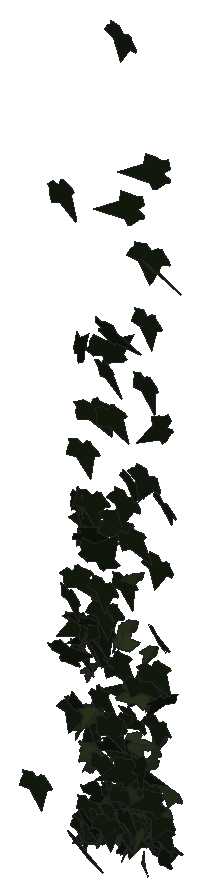
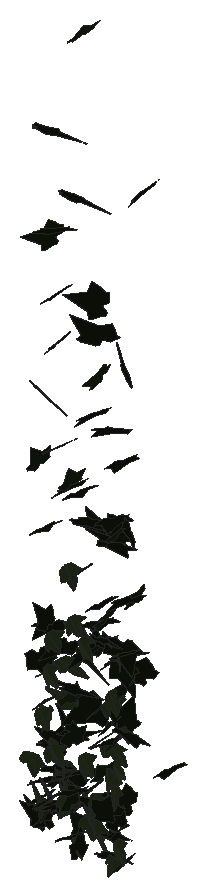
# SketchUp Ruby script. Lengths in inches.
U = 1.inch
M = Sketchup.active_model
def pt(a) = Geom::Point3d.new(a.map { |v| v * U })
def face(e, loops, mat)
  f = e.add_face(loops[0].map { |a| pt(a) })
  loops[1..].each { |l| e.add_face(l.map { |a| pt(a) }).erase! }
  f.material = f.back_material = mat if mat
  f
end
# faces: each face lists its corners as indices into pts; further lists are holes
def faces(e, pts, list, mat = nil) = list.each { |f| face(e, (f[0].is_a?(Array) ? f : [f]).map { |l| l.map { |i| pts[i] } }, mat) }
# xy, xz, yz: faces in a plane at the given z, y or x. An outline is a flat list of corners, or four numbers for a rectangle; further outlines are holes
def ring(l) = l.size == 4 ? [[l[0], l[1]], [l[2], l[1]], [l[2], l[3]], [l[0], l[3]]] : l.each_slice(2).to_a
def flat(e, list, mat, &to3) = list.each { |f| face(e, (f[0].is_a?(Array) ? f : [f]).map { |l| ring(l).map { |u, v| to3.(u, v) } }, mat) }
def xy(e, z, list, mat = nil) = flat(e, list, mat) { |x, y| [x, y, z] }
def xz(e, y, list, mat = nil) = flat(e, list, mat) { |x, z| [x, y, z] }
def yz(e, x, list, mat = nil) = flat(e, list, mat) { |y, z| [x, y, z] }
def lines(e, pts, list) = list.each { |a, b| e.add_line(pt(pts[a]), pt(pts[b])) }
# prism: a flat outline (further loops are holes) pulled along v
def prism(e, loops, v, mat = nil)
  f = face(e, loops, mat); d = Geom::Vector3d.new(v.map { |x| x * U })
  f.pushpull(f.normal.samedirection?(d) ? d.length : -d.length)
end
def box(e, o, s, mat = nil) = prism(e, [[o, [o[0] + s[0], o[1], o[2]], [o[0] + s[0], o[1] + s[1], o[2]], [o[0], o[1] + s[1], o[2]]]], [0, 0, s[2]], mat)
def at(x, y, z, deg = 0) = Geom::Transformation.translation(pt([x, y, z])) * Geom::Transformation.rotation(ORIGIN, Z_AXIS, deg.degrees)
def axes(o, x, y, z) = Geom::Transformation.new([*x, 0, *y, 0, *z, 0, *pt(o).to_a, 1])
def part(name) = M.definitions.add(name)
# library, detail: a bought-in or finely detailed component or shape, given as its bounding box
def library(name, o, s) = part(name).tap { |d| box(d.entities, o, s) }
def detail(e, o, s) = box(e.add_group.entities, o, s)
def put(e, d, t, mat = nil) = e.add_instance(d, t).tap { |i| i.material = mat if mat }
def group(e, t, mat = nil) = e.add_group.tap { |g| g.transformation = t; g.material = mat if mat }.entities
root = M.entities
M.materials.add("1026 AP 7946 SUNNY SIDE UP").color = [254, 231, 186]
M.materials.add("efeu1").color = [18, 25, 13]
M.materials.add("efeu2").color = [43, 57, 29]
c1 = part("ivyleaf_9")
p = [[1.54,2.16,1.25],[1.36,2.04,1.19],[-0.21,0.99,0.68],[-0.71,1.11,0.82],[-0.85,0.86,0.67],[-0.8,0.17,0.21],
  [-0.9,-0.01,0.1],[-0.67,-0.16,-0.02],[-0.08,-0.08,-0.05],[-0.03,-0.6,-0.4],[0.65,-0.88,-0.66],[0.83,-0.6,-0.49],
  [1.29,-0.42,-0.43],[1.8125,-0.07,-0.26],[1.21,0.44,0.15]]
faces(c1.entities,p,[[0,1,2,3,4,5,6,7,8,9,10,11,12,13,14]],"efeu1")
c2 = part("ivyleaf_10")
p = [[0,0.5,-0.03],[-0.0625,2.02,-0.43],[-0.19,2.01,-0.46],[-0.54,1.05,-0.29],[-0.52,0.625,-0.18],[-0.83,0.76,-0.28],
  [-1.16,0.64,-0.33],[-1.15,0.33,-0.24],[-0.77,-0.39,0.02],[-0.3,-0.51,0.16],[0.04,-0.48,0.23],[-0.02,2.01,-0.4375],
  [-0.06,2.01,-0.43],[0.04,-0.49,0.23],[0.67,-0.49,0.14],[1.38,0.36,-0.2],[1.375,0.51,-0.24],[0.81,0.65,-0.19],
  [0.62,0.59,-0.15],[0.6,1.09,-0.28],[0.5,1.23,-0.31]]
faces(c2.entities,p,[[0,1,2,3,4,5,6,7,8,9,10],[11,12,0,13,14,15,16,17,18,19,20]],"efeu2")
put(root,c1,axes([128.56,209.27,294.41],[-0.04738,-0.42398,-0.02706],[0.01155,0.0234,-0.4377],[0.66762,-0.03049,0.00565]),"1026 AP 7946 SUNNY SIDE UP")
put(root,c1,axes([128.95,211.87,300.18],[-0.0411,0.3727,-0.15385],[0.00882,-0.15142,-0.38575],[-0.63252,-0.02633,0.00462]),"1026 AP 7946 SUNNY SIDE UP")
put(root,c1,axes([128.49,211.98,306.7],[-0.12389,-0.05519,-0.4269],[0.64213,-0.09887,-0.06706],[-0.13826,-0.40974,0.0711]),"1026 AP 7946 SUNNY SIDE UP")
put(root,c1,axes([129.01,211.92,300.68],[-0.41349,-0.17235,0.25958],[-0.22045,-0.22861,-0.31197],[0.42783,-0.28438,0.09012]),"1026 AP 7946 SUNNY SIDE UP")
put(root,c1,axes([128.59,210.75,321.9],[0.2203,-0.41557,-0.15776],[-0.0865,0.14055,-0.45091],[0.68972,0.15036,-0.00616]),"1026 AP 7946 SUNNY SIDE UP")
put(root,c1,axes([128.54,212.12,299.43],[0.26085,-0.35707,0.08476],[0.0309,-0.08374,-0.40572],[0.57607,0.16618,-0.01662]),"1026 AP 7946 SUNNY SIDE UP")
put(root,c1,axes([129.04,211.73,301.09],[0.35806,0.18051,-0.29653],[-0.32642,-0.20194,-0.29977],[-0.42465,0.30744,-0.0196]),"1026 AP 7946 SUNNY SIDE UP")
put(root,c1,axes([128.72,211.84,313.61],[-0.15711,0.27646,0.35608],[0.04417,-0.34808,0.2945],[0.69263,0.08491,0.06199]),"1026 AP 7946 SUNNY SIDE UP")
put(root,c1,axes([128.93,211.61,296.98],[-0.53194,-0.14995,-0.15935],[0.25623,0.00787,-0.37704],[0.22011,-0.37155,0.05379]),"1026 AP 7946 SUNNY SIDE UP")
put(root,c1,axes([128.47,211.0625,299.54],[0.0785,-0.05328,0.42746],[0.58272,-0.1889,-0.07198],[0.30621,0.37314,0.02738]),"1026 AP 7946 SUNNY SIDE UP")
put(root,c2,axes([128.98,212.14,295.52],[0.19769,-0.27738,0.24056],[0.13137,-0.22005,-0.3148],[0.55643,0.1505,-0.01115]),"1026 AP 7946 SUNNY SIDE UP")
put(root,c1,axes([128.73,211.59,303.26],[0.13865,-0.32995,-0.24227],[0.09356,0.24678,-0.33496],[0.62848,0.03606,0.10331]),"1026 AP 7946 SUNNY SIDE UP")
put(root,c1,axes([128.83,211.97,291.09],[0.02901,-0.34255,0.15185],[0.02884,-0.14852,-0.35413],[0.58688,0.02423,0.0099]),"1026 AP 7946 SUNNY SIDE UP")
put(root,c2,axes([129.1,211.97,291.82],[0.0718,-0.36619,0.07213],[0.00868,-0.07196,-0.38057],[0.58679,0.04587,-0.0032]),"1026 AP 7946 SUNNY SIDE UP")
put(root,c2,axes([129.27,212.14,298.76],[-0.06553,-0.38482,0.04777],[-0.00155,-0.04873,-0.39902],[0.60989,-0.04147,0.00412]),"1026 AP 7946 SUNNY SIDE UP")
put(root,c2,axes([129.26,211.96,294.35],[0.05907,-0.35901,-0.11101],[0.04235,0.10856,-0.36932],[0.58695,0.0283,0.03782]),"1026 AP 7946 SUNNY SIDE UP")
put(root,c2,axes([129.3,211.55,300.43],[0.13711,-0.37617,-0.10241],[0.03993,0.10499,-0.39423],[0.60963,0.07772,0.04885]),"1026 AP 7946 SUNNY SIDE UP")
put(root,c1,axes([129.41,212.04,305.75],[-0.54344,-0.22435,-0.02722],[0.07006,-0.02271,-0.42227],[0.34799,-0.34578,0.04251]),"1026 AP 7946 SUNNY SIDE UP")
put(root,c1,axes([129.36,211.19,297.07],[0.48866,-0.2195,0.15292],[-0.15361,0.1198,0.39064],[-0.38848,-0.32347,0.03789]),"1026 AP 7946 SUNNY SIDE UP")
put(root,c1,axes([129.18,211.55,309.45],[-0.04786,-0.4147,-0.08666],[0.0314,0.08047,-0.42766],[0.66388,-0.0337,0.01398]),"1026 AP 7946 SUNNY SIDE UP")
put(root,c1,axes([129.12,210.76,302.8],[0.17656,-0.36619,0.1307],[0.02009,-0.13068,-0.39453],[0.61013,0.11027,-0.02483]),"1026 AP 7946 SUNNY SIDE UP")
put(root,c1,axes([129.28,211.83,292.41],[0.02982,-0.371,-0.00111],[-0.00318,-0.00113,-0.3827],[0.58336,0.01896,-0.00203]),"1026 AP 7946 SUNNY SIDE UP")
put(root,c1,axes([129.32,211.98,306.89],[-0.15319,-0.39237,-0.12694],[0.05365,0.11619,-0.41578],[0.6434,-0.10311,0.00444]),"1026 AP 7946 SUNNY SIDE UP")
put(root,c2,axes([129.6,211.54,294.83],[-0.46446,0.25585,0.09748],[-0.13842,0.04034,-0.40142],[-0.40515,-0.30709,0.0254]),"1026 AP 7946 SUNNY SIDE UP")
put(root,c2,axes([129.51,211.69,291.04],[-0.12512,-0.31163,-0.18014],[0.10844,0.16054,-0.32949],[0.54993,-0.10256,0.02398]),"1026 AP 7946 SUNNY SIDE UP")
put(root,c1,axes([129.19,212.1,311.16],[-0.00387,-0.36821,-0.22372],[0.25765,0.19775,-0.34955],[0.61903,-0.08461,0.14409]),"1026 AP 7946 SUNNY SIDE UP")
put(root,c1,axes([129.8,211.91,291.22],[-0.50084,-0.11864,0.12061],[-0.14088,-0.09275,-0.34649],[0.22188,-0.32668,0.05226]),"1026 AP 7946 SUNNY SIDE UP")
put(root,c1,axes([129.29,211.91,300.42],[0.12777,-0.42032,0.03332],[-0.00222,-0.03564,-0.44116],[0.66316,0.08087,-0.00789]),"1026 AP 7946 SUNNY SIDE UP")
put(root,c1,axes([129.29,211.74,306.08],[0.21573,-0.38408,0.00639],[-0.01423,-0.01213,-0.42004],[0.60391,0.13692,-0.01218]),"1026 AP 7946 SUNNY SIDE UP")
put(root,c2,axes([129.58,211.98,295.01],[0.10351,-0.35332,-0.12357],[0.04067,0.12382,-0.36652],[0.58429,0.05397,0.04741]),"1026 AP 7946 SUNNY SIDE UP")
put(root,c1,axes([129.61,212.32,296.58],[-0.23444,-0.33015,0.13216],[-0.03776,-0.13147,-0.37265],[0.55674,-0.14794,0.03037]),"1026 AP 7946 SUNNY SIDE UP")
put(root,c2,axes([129.76,210.91,296.74],[0.0618,-0.37587,0.09438],[-0.00164,-0.09433,-0.38973],[0.60912,0.03788,-0.01062]),"1026 AP 7946 SUNNY SIDE UP")
put(root,c1,axes([129.49,212.23,302.35],[0.25846,-0.36497,-0.00442],[-0.00832,0.00005,-0.41233],[0.57383,0.16439,-0.00399]),"1026 AP 7946 SUNNY SIDE UP")
put(root,c1,axes([129.87,211.6,292.03],[-0.50144,-0.19099,-0.07715],[0.12299,0.01261,-0.38172],[0.29754,-0.32709,0.02776]),"1026 AP 7946 SUNNY SIDE UP")
put(root,c1,axes([130.01,211.95,301.1],[-0.59866,-0.06598,-0.04487],[0.0782,-0.0357,-0.39576],[0.09622,-0.3815,0.04247]),"1026 AP 7946 SUNNY SIDE UP")
put(root,c1,axes([129.78,211.6,296.01],[-0.15645,-0.17918,0.35808],[-0.09271,-0.34872,-0.20403],[0.6093,-0.09907,0.0609]),"1026 AP 7946 SUNNY SIDE UP")
put(root,c2,axes([130.3125,210.95,295.56],[-0.46905,-0.0013,0.25786],[-0.37344,-0.12153,-0.29294],[0.12432,-0.36996,0.09292]),"1026 AP 7946 SUNNY SIDE UP")
put(root,c1,axes([129.9,212.1,302.85],[-0.09306,-0.39545,0.04862],[-0.00544,-0.04947,-0.41219],[0.62662,-0.05916,0.00364]),"1026 AP 7946 SUNNY SIDE UP")
put(root,c1,axes([129.95,211.4,296.86],[0.01971,-0.3927,0.20393],[-0.01234,-0.20043,-0.40573],[0.69297,0.0076,-0.01302]),"1026 AP 7946 SUNNY SIDE UP")
put(root,c2,axes([130.27,212.13,292.5625],[-0.56982,-0.0095,0.02651],[-0.03603,-0.08384,-0.36402],[0.02386,-0.35349,0.08344]),"1026 AP 7946 SUNNY SIDE UP")
put(root,c1,axes([129.6875,211.64,293],[0.12614,0.00816,0.41124],[0.61037,-0.0967,-0.0789],[0.14665,0.39547,-0.02533]),"1026 AP 7946 SUNNY SIDE UP")
put(root,c1,axes([130.09,212.02,301.89],[-0.21394,-0.40495,-0.05351],[0.06395,0.0386,-0.43905],[0.63831,-0.13959,0.02606]),"1026 AP 7946 SUNNY SIDE UP")
put(root,c1,axes([129.77,210.84,305.81],[0.17861,0.12411,-0.39042],[0.33621,0.31453,0.17365],[0.53054,-0.24111,0.02139]),"1026 AP 7946 SUNNY SIDE UP")
put(root,c1,axes([129.93,212,313.3125],[0.34066,-0.37409,-0.00122],[-0.02292,-0.00953,-0.44504],[0.58777,0.21644,-0.01665]),"1026 AP 7946 SUNNY SIDE UP")
put(root,c1,axes([130.01,211.53,298.02],[0.30948,-0.32183,-0.19003],[-0.11239,0.1699,-0.38679],[0.5709,0.20791,0.02687]),"1026 AP 7946 SUNNY SIDE UP")
put(root,c2,axes([130.37,210.87,297.45],[-0.21891,-0.25465,0.26988],[-0.02146,-0.27799,-0.28591],[0.5757,-0.10719,0.09197]),"1026 AP 7946 SUNNY SIDE UP")
put(root,c1,axes([130.02,211.74,294.74],[0.0298,-0.3344,0.23073],[0.10208,-0.22065,-0.34343],[0.62625,0.05187,0.045]),"1026 AP 7946 SUNNY SIDE UP")
put(root,c2,axes([130.32,211.55,291.5],[0.2564,-0.33559,0.04353],[0.00453,-0.04764,-0.3842],[0.53222,0.16208,-0.0177]),"1026 AP 7946 SUNNY SIDE UP")
put(root,c1,axes([130.02,210.84,292.08],[0.02259,-0.10963,0.42743],[0.24033,-0.38727,-0.11297],[0.63154,0.15129,0.0277]),"1026 AP 7946 SUNNY SIDE UP")
put(root,c1,axes([130.16,211.7,300.99],[-0.32341,-0.08176,-0.36657],[0.57157,-0.01374,-0.21357],[0.0453,-0.41036,0.07768]),"1026 AP 7946 SUNNY SIDE UP")
put(root,c2,axes([130.43,211.99,292.58],[0.21,-0.34816,0.06295],[0.01652,-0.0635,-0.38431],[0.55612,0.13336,-0.01235]),"1026 AP 7946 SUNNY SIDE UP")
put(root,c2,axes([130.65,212.17,295.375],[-0.01764,-0.35874,0.10209],[-0.00956,-0.10099,-0.37033],[0.58599,-0.01245,-0.00297]),"1026 AP 7946 SUNNY SIDE UP")
put(root,c2,axes([130.63,211.51,293.3],[-0.07246,-0.36994,-0.12874],[0.06564,0.11832,-0.38247],[0.60942,-0.05673,0.02589]),"1026 AP 7946 SUNNY SIDE UP")
put(root,c1,axes([130.4,211.27,300.18],[-0.10587,-0.25855,0.32156],[0.11536,-0.32038,-0.25776],[0.62859,0.01525,0.10146]),"1026 AP 7946 SUNNY SIDE UP")
put(root,c1,axes([130.36,211.83,311.36],[0.12821,-0.39152,-0.17854],[0.05752,0.17993,-0.40518],[0.66937,0.05953,0.06902]),"1026 AP 7946 SUNNY SIDE UP")
put(root,c2,axes([130.7,212.21,300.7],[0.13445,-0.36547,0.13187],[0.02507,-0.12978,-0.38719],[0.60947,0.08596,-0.01316]),"1026 AP 7946 SUNNY SIDE UP")
put(root,c1,axes([130.95,211.97,306.27],[-0.57146,-0.1697,0.10968],[-0.12904,-0.07726,-0.41217],[0.28825,-0.37102,0.03294]),"1026 AP 7946 SUNNY SIDE UP")
put(root,c2,axes([130.8125,212.12,295.25],[0.07368,-0.37363,-0.02803],[0.01727,0.02664,-0.3875],[0.58857,0.04599,0.01488]),"1026 AP 7946 SUNNY SIDE UP")
put(root,c1,axes([130.57,212.44,329.09],[-0.09441,-0.40677,0.25402],[0.04821,-0.25362,-0.4209],[0.74828,-0.03498,0.05916]),"1026 AP 7946 SUNNY SIDE UP")
put(root,c1,axes([130.7,210.63,304.99],[-0.44244,0.14755,0.36759],[0.48972,-0.17248,0.32626],[0.35681,0.4197,0.00802]),"1026 AP 7946 SUNNY SIDE UP")
put(root,c1,axes([130.6,211.2,314.47],[-0.23703,0.00311,0.44982],[0.68509,0.03134,0.15492],[-0.04499,0.46085,-0.01086]),"1026 AP 7946 SUNNY SIDE UP")
put(root,c1,axes([131.5,212.19,321.22],[-0.60877,0.10661,0.22234],[-0.36168,-0.0471,-0.40251],[-0.10867,-0.44045,0.0941]),"1026 AP 7946 SUNNY SIDE UP")
put(root,c1,axes([130.8,211.46,293.7],[0.09131,-0.37887,0.07008],[0.00921,-0.07009,-0.39524],[0.6058,0.05817,-0.00455]),"1026 AP 7946 SUNNY SIDE UP")
put(root,c1,axes([131.09,211.98,290.85],[0.1084,0.23171,0.30612],[-0.28636,-0.24248,0.23796],[0.51684,-0.18295,0.06764]),"1026 AP 7946 SUNNY SIDE UP")
put(root,c1,axes([130.65,209.33,292.08],[0.42967,-0.30291,0.24829],[0.20602,-0.20744,-0.41986],[0.57453,0.30092,-0.03513]),"1026 AP 7946 SUNNY SIDE UP")
put(root,c1,axes([131.45,211.25,292.79],[-0.52807,-0.13084,0.15549],[-0.19992,-0.08956,-0.37014],[0.24338,-0.35745,0.03333]),"1026 AP 7946 SUNNY SIDE UP")
put(root,c1,axes([130.9375,210.625,295.58],[0.07863,-0.391,-0.00516],[0.0032,0.00307,-0.40606],[0.61481,0.04999,0.00277]),"1026 AP 7946 SUNNY SIDE UP")
put(root,c2,axes([130.85,211.2,292.09],[0.37398,-0.00605,0.28405],[0.42748,-0.05635,-0.24316],[0.07325,0.35977,-0.03116]),"1026 AP 7946 SUNNY SIDE UP")
put(root,c1,axes([131.68,212.07,298.33],[-0.44467,0.06475,0.26052],[-0.40555,-0.01532,-0.2936],[-0.05961,-0.37882,0.05412]),"1026 AP 7946 SUNNY SIDE UP")
put(root,c2,axes([131.26,211.62,300.73],[0.61098,-0.0298,0.08601],[-0.11803,0.09049,0.39288],[-0.07464,-0.38703,0.08283]),"1026 AP 7946 SUNNY SIDE UP")
put(root,c1,axes([131.01,211.4,299.99],[0.16176,-0.32987,-0.29985],[-0.05833,0.28943,-0.35202],[0.68732,0.1022,0.04069]),"1026 AP 7946 SUNNY SIDE UP")
put(root,c1,axes([131.18,211.97,307.48],[-0.18367,-0.39982,0.08641],[-0.0128,-0.0873,-0.42929],[0.64298,-0.11595,0.01614]),"1026 AP 7946 SUNNY SIDE UP")
put(root,c2,axes([131.34,212.1,301.48],[-0.09437,-0.34304,0.18757],[0.07008,-0.19103,-0.35299],[0.60808,-0.03122,0.06979]),"1026 AP 7946 SUNNY SIDE UP")
put(root,c2,axes([131.39,211.84,291.09],[0.24145,-0.312,0.09256],[0.04078,-0.08924,-0.3584],[0.50968,0.15495,-0.01517]),"1026 AP 7946 SUNNY SIDE UP")
put(root,c1,axes([130.81,210.93,315.84],[0.50145,-0.17304,0.32636],[0.38744,-0.20634,-0.3717],[0.41665,0.40013,-0.04714]),"1026 AP 7946 SUNNY SIDE UP")
put(root,c1,axes([131.3,212.14,293.71],[-0.21536,-0.33943,-0.03732],[0.08486,0.01494,-0.37422],[0.52969,-0.1404,0.04478]),"1026 AP 7946 SUNNY SIDE UP")
put(root,c1,axes([131.2,211.78,303.72],[0.08621,-0.40175,-0.00956],[-0.01285,0.00595,-0.41762],[0.63169,0.05495,-0.00719]),"1026 AP 7946 SUNNY SIDE UP")
put(root,c1,axes([131.19,212.35,308.07],[-0.04571,-0.30678,0.28953],[0.10675,-0.28317,-0.31095],[0.64732,0.02504,0.07172]),"1026 AP 7946 SUNNY SIDE UP")
put(root,c2,axes([131.55,212.15,303.82],[-0.13651,-0.38127,0.07104],[-0.02124,-0.06986,-0.40324],[0.60949,-0.08783,0.00186]),"1026 AP 7946 SUNNY SIDE UP")
put(root,c1,axes([131.34,210.59,292.74],[-0.11337,-0.38327,-0.02404],[0.01431,0.01981,-0.40162],[0.60341,-0.07248,0.00501]),"1026 AP 7946 SUNNY SIDE UP")
put(root,c1,axes([131.5,212.13,291.52],[-0.20331,-0.33183,0.07806],[0.02829,-0.08959,-0.36404],[0.53512,-0.12134,0.04891]),"1026 AP 7946 SUNNY SIDE UP")
put(root,c1,axes([131.5,212.38,293.75],[-0.11951,-0.34452,0.13818],[0.01255,-0.14041,-0.36243],[0.58231,-0.06768,0.03617]),"1026 AP 7946 SUNNY SIDE UP")
put(root,c1,axes([131.42,211.19,294.15],[0.0813,-0.29555,-0.24866],[0.02194,0.2432,-0.30441],[0.59794,0.03126,0.04498]),"1026 AP 7946 SUNNY SIDE UP")
put(root,c1,axes([131.33,212.21,293.13],[0.1232,-0.25371,0.25397],[0.15794,-0.22768,-0.27402],[0.535,0.12564,0.02241]),"1026 AP 7946 SUNNY SIDE UP")
put(root,c1,axes([131.3,211.41,291.68],[0.10496,-0.24554,0.31351],[0.21758,-0.27542,-0.26061],[0.57689,0.14855,0.04126]),"1026 AP 7946 SUNNY SIDE UP")
put(root,c1,axes([131.52,211.51,292.68],[0.1159,-0.36474,0.07348],[0.01482,-0.07297,-0.38374],[0.58483,0.07413,-0.00484]),"1026 AP 7946 SUNNY SIDE UP")
put(root,c1,axes([131.46,210.29,296.72],[0.60519,0.22081,0.1819],[0.26166,0.06157,-0.4559],[-0.35788,0.41843,-0.02572]),"1026 AP 7946 SUNNY SIDE UP")
put(root,c2,axes([131.79,211.88,293],[-0.21772,-0.31505,-0.13241],[0.12332,0.1035,-0.35272],[0.51953,-0.1566,0.02824]),"1026 AP 7946 SUNNY SIDE UP")
put(root,c1,axes([131.68,211.25,292.61],[-0.04532,-0.36531,-0.00168],[-0.00573,-0.00016,-0.37749],[0.57439,-0.02882,-0.0039]),"1026 AP 7946 SUNNY SIDE UP")
put(root,c1,axes([131.6,211.72,295.76],[-0.11602,-0.17764,0.38535],[0.21113,-0.37067,-0.15582],[0.61746,0.09337,0.12569]),"1026 AP 7946 SUNNY SIDE UP")
put(root,c1,axes([131.7,211.39,293.47],[-0.11795,-0.01241,0.39459],[0.50554,0.2105,0.07311],[-0.32814,0.32876,-0.0292]),"1026 AP 7946 SUNNY SIDE UP")
put(root,c1,axes([132.36,211.12,295.44],[-0.39836,-0.30622,-0.12282],[-0.15216,-0.07205,0.40803],[-0.49276,0.2698,-0.02671]),"1026 AP 7946 SUNNY SIDE UP")
put(root,c1,axes([132.25,211.35,293.84],[-0.42887,0.24519,-0.04366],[0.01989,-0.0512,-0.37691],[-0.39112,-0.27145,0.02871]),"1026 AP 7946 SUNNY SIDE UP")
put(root,c2,axes([131.99,211.76,294.14],[0.09368,-0.34735,-0.11434],[0.02774,0.11309,-0.36062],[0.57177,0.05142,0.03623]),"1026 AP 7946 SUNNY SIDE UP")
put(root,c1,axes([131.72,211.2,292.95],[0.19784,-0.3448,-0.02013],[-0.0113,0.0161,-0.37802],[0.54275,0.12602,-0.00053]),"1026 AP 7946 SUNNY SIDE UP")
put(root,c1,axes([131.96,211.6,297.4],[-0.258,-0.1951,0.32285],[0.05153,-0.35032,-0.20832],[0.57965,-0.05569,0.16222]),"1026 AP 7946 SUNNY SIDE UP")
put(root,c2,axes([132.41,211.27,298.87],[0.36302,0.00508,-0.33289],[-0.50681,-0.02582,-0.23779],[-0.03767,0.39632,-0.0089]),"1026 AP 7946 SUNNY SIDE UP")
put(root,c2,axes([132.36,211.12,294.03],[-0.43202,0.14037,0.21258],[-0.3284,0.03655,-0.31309],[-0.21292,-0.34118,0.05157]),"1026 AP 7946 SUNNY SIDE UP")
put(root,c1,axes([131.99,212.19,293.91],[-0.09461,-0.27014,0.24524],[0.10835,-0.24701,-0.27054],[0.55732,0.00217,0.09423]),"1026 AP 7946 SUNNY SIDE UP")
put(root,c2,axes([132.32,212.2,295.23],[-0.17512,-0.30961,0.17727],[-0.05958,-0.17078,-0.33936],[0.55513,-0.116,0.0195]),"1026 AP 7946 SUNNY SIDE UP")
put(root,c1,axes([132.32,212.25,293.86],[-0.36428,-0.1873,0.22272],[-0.10986,-0.23401,-0.28595],[0.43746,-0.21473,0.11366]),"1026 AP 7946 SUNNY SIDE UP")
put(root,c2,axes([132.34,211.85,294.13],[0.19536,-0.33463,-0.09804],[-0.07155,0.08252,-0.36698],[0.54153,0.13162,-0.01312]),"1026 AP 7946 SUNNY SIDE UP")
put(root,c2,axes([132.29,212.28,300.51],[-0.06814,-0.35363,0.18299],[0.03871,-0.18275,-0.36558],[0.62247,-0.02735,0.04277]),"1026 AP 7946 SUNNY SIDE UP")
put(root,c2,axes([132.375,212.14,295.42],[0.19479,-0.36472,0.01671],[-0.0088,-0.02121,-0.39675],[0.57415,0.12341,-0.01175]),"1026 AP 7946 SUNNY SIDE UP")
put(root,c1,axes([132.22,212.27,319.42],[-0.29124,-0.40681,-0.04792],[0.15298,0.00335,-0.45171],[0.62498,-0.19039,0.08824]),"1026 AP 7946 SUNNY SIDE UP")
put(root,c1,axes([132.18,212.09,316.36],[-0.00171,-0.43843,0.05736],[-0.00179,-0.05817,-0.45201],[0.69543,-0.00123,-0.00102]),"1026 AP 7946 SUNNY SIDE UP")
put(root,c1,axes([132.2,211.68,292.66],[-0.13021,-0.36025,-0.18738],[0.12615,0.16517,-0.37792],[0.62043,-0.10919,0.03751]),"1026 AP 7946 SUNNY SIDE UP")
put(root,c1,axes([132.48,211.88,294.28],[-0.38153,-0.28009,0.01229],[0.01457,-0.02588,-0.38112],[0.44069,-0.24164,0.02324]),"1026 AP 7946 SUNNY SIDE UP")
put(root,c1,axes([132.42,212.34,298.89],[-0.26181,-0.3108,0.17779],[0.01354,-0.19589,-0.35242],[0.56018,-0.14052,0.09161]),"1026 AP 7946 SUNNY SIDE UP")
put(root,c1,axes([132.44,211.78,309.03],[-0.22112,-0.36536,0.1807],[-0.00429,-0.18696,-0.39983],[0.63868,-0.12775,0.05987]),"1026 AP 7946 SUNNY SIDE UP")
put(root,c1,axes([133.08,211.9,323.63],[-0.60529,0.08191,0.25118],[-0.40145,-0.07535,-0.39036],[-0.04303,-0.44914,0.10851]),"1026 AP 7946 SUNNY SIDE UP")
put(root,c1,axes([133.01,209.49,298.35],[-0.47218,0.33157,0.04709],[-0.09129,0.00632,-0.45909],[-0.51792,-0.30341,0.03799]),"1026 AP 7946 SUNNY SIDE UP")
put(root,c2,axes([132.67,212,298.65],[0.08859,-0.36316,0.14667],[0.0109,-0.14498,-0.37916],[0.61444,0.05493,-0.01442]),"1026 AP 7946 SUNNY SIDE UP")
put(root,c1,axes([132.4375,211.68,292.45],[0.00673,-0.33956,-0.15949],[0.04932,0.15269,-0.34755],[0.58347,-0.00899,0.03122]),"1026 AP 7946 SUNNY SIDE UP")
put(root,c1,axes([132.45,211.13,299.69],[0.09246,-0.20075,-0.3768],[0.02396,0.36903,-0.20462],[0.65404,0.01486,0.06077]),"1026 AP 7946 SUNNY SIDE UP")
put(root,c1,axes([132.45,210.56,306.8],[0.19279,-0.3532,-0.20543],[0.02795,0.21077,-0.3759],[0.63562,0.09786,0.07884]),"1026 AP 7946 SUNNY SIDE UP")
put(root,c1,axes([132.52,211.5,313.75],[0.14314,-0.43381,0.04317],[-0.00823,-0.04641,-0.45667],[0.68563,0.09001,-0.0145]),"1026 AP 7946 SUNNY SIDE UP")
put(root,c1,axes([132.57,209.05,298.7],[0.13152,-0.39834,-0.22428],[-0.07264,0.21044,-0.41808],[0.70837,0.09554,-0.00123]),"1026 AP 7946 SUNNY SIDE UP")
put(root,c1,axes([133.24,209.58,296.26],[-0.62993,0.15296,0.07582],[-0.126,-0.00663,-0.4404],[-0.23463,-0.40711,0.03294]),"1026 AP 7946 SUNNY SIDE UP")
put(root,c1,axes([132.46,212.34,301.16],[0.11821,-0.17498,0.36072],[0.19641,-0.32825,-0.19798],[0.58479,0.14562,-0.00642]),"1026 AP 7946 SUNNY SIDE UP")
put(root,c1,axes([132.63,212.18,292.83],[0.07759,-0.35727,-0.05532],[-0.00401,0.0518,-0.37122],[0.5676,0.0492,0.00494]),"1026 AP 7946 SUNNY SIDE UP")
put(root,c1,axes([132.37,212.02,318.9375],[0.49136,-0.29868,0.11662],[0.19846,-0.03255,-0.44098],[0.46241,0.33135,0.06534]),"1026 AP 7946 SUNNY SIDE UP")
put(root,c1,axes([132.38,211.39,295.12],[0.24704,-0.12024,0.35254],[0.38813,-0.23882,-0.20419],[0.41928,0.29193,-0.0187]),"1026 AP 7946 SUNNY SIDE UP")
put(root,c2,axes([132.85,212.01,293.35],[0.40507,-0.2591,0.06944],[0.05202,-0.06408,-0.37613],[0.41833,0.25885,-0.02047]),"1026 AP 7946 SUNNY SIDE UP")
put(root,c1,axes([132.75,212.1,297.28],[-0.08804,-0.3705,0.15928],[0.02711,-0.16029,-0.38498],[0.63196,-0.04474,0.0387]),"1026 AP 7946 SUNNY SIDE UP")
put(root,c1,axes([133.27,211.95,311.58],[-0.63606,0.18747,-0.047],[0.03787,-0.05854,-0.45753],[-0.30141,-0.40297,0.04169]),"1026 AP 7946 SUNNY SIDE UP")
put(root,c2,axes([132.47,210.77,296.86],[0.1296,-0.05904,-0.39573],[0.60174,-0.05419,0.09294],[-0.10355,-0.38879,0.04477]),"1026 AP 7946 SUNNY SIDE UP")
put(root,c1,axes([132.75,210.83,296.07],[-0.27351,-0.0356,-0.38792],[0.58603,-0.08551,-0.16962],[-0.09952,-0.40569,0.0673]),"1026 AP 7946 SUNNY SIDE UP")
put(root,c2,axes([133,211.78,292.36],[-0.21948,-0.32049,-0.11595],[0.08757,0.09646,-0.35934],[0.52593,-0.1498,0.01145]),"1026 AP 7946 SUNNY SIDE UP")
put(root,c2,axes([133.0625,211.99,296.625],[-0.04171,-0.36542,0.09586],[-0.00861,-0.09498,-0.37799],[0.59367,-0.02705,0.00125]),"1026 AP 7946 SUNNY SIDE UP")
put(root,c2,axes([133.09,210.55,292.72],[0.29481,-0.34359,0.04018],[0.00518,-0.0448,-0.40305],[0.54407,0.18661,-0.01793]),"1026 AP 7946 SUNNY SIDE UP")
put(root,c2,axes([133.03,211.47,296.48],[0.17644,-0.29988,-0.25578],[0.10632,0.26784,-0.30231],[0.60113,0.04064,0.12854]),"1026 AP 7946 SUNNY SIDE UP")
put(root,c1,axes([133.06,212.1,291.73],[-0.18895,-0.09448,0.34492],[-0.0859,-0.34524,-0.12239],[0.54105,-0.08781,0.10103]),"1026 AP 7946 SUNNY SIDE UP")
put(root,c1,axes([133.07,211.83,305.12],[-0.16625,-0.37536,0.09806],[-0.02346,-0.09685,-0.40213],[0.60927,-0.10615,0.01127]),"1026 AP 7946 SUNNY SIDE UP")
put(root,c2,axes([133.33,212.06,293.11],[0.35472,-0.28193,-0.06593],[-0.04666,0.05613,-0.37145],[0.45162,0.22723,0.01341]),"1026 AP 7946 SUNNY SIDE UP")
put(root,c2,axes([133.51,210.21,291.67],[-0.20556,0.17366,0.3096],[-0.3075,0.22719,-0.22229],[-0.44928,-0.23495,0.01048]),"1026 AP 7946 SUNNY SIDE UP")
put(root,c1,axes([133.52,211.52,298.95],[-0.06544,0.3378,-0.25135],[0.02626,-0.24558,-0.35189],[-0.65647,-0.0435,0.01098]),"1026 AP 7946 SUNNY SIDE UP")
put(root,c1,axes([132.92,212.02,291.78],[0.18184,-0.148,0.33638],[0.33016,-0.25121,-0.19488],[0.45838,0.23965,0.00693]),"1026 AP 7946 SUNNY SIDE UP")
put(root,c1,axes([133.13,211.23,300.43],[-0.02064,-0.30361,-0.27191],[0.07023,0.25962,-0.31047],[0.62688,-0.03909,0.02583]),"1026 AP 7946 SUNNY SIDE UP")
put(root,c2,axes([133.57,211.91,294.37],[-0.56128,0.07989,0.08537],[-0.14309,-0.03291,-0.37339],[-0.10999,-0.36487,0.05012]),"1026 AP 7946 SUNNY SIDE UP")
put(root,c1,axes([133.42,211.6,293.23],[-0.27806,-0.30305,0.1164],[-0.0182,-0.12468,-0.35847],[0.50918,-0.16995,0.05075]),"1026 AP 7946 SUNNY SIDE UP")
put(root,c1,axes([133.24,211.64,292.59],[0.12847,-0.35419,-0.11743],[0.00372,0.11515,-0.37276],[0.58409,0.07717,0.0282]),"1026 AP 7946 SUNNY SIDE UP")
put(root,c1,axes([133.1875,211.63,291.31],[-0.04457,0.05181,0.39871],[0.34461,-0.31869,0.05867],[0.50761,0.22091,-0.00482]),"1026 AP 7946 SUNNY SIDE UP")
put(root,c1,axes([133.86,210.73,294.43],[-0.39724,-0.08343,0.27051],[-0.31834,-0.18633,-0.26227],[0.29489,-0.31353,0.08127]),"1026 AP 7946 SUNNY SIDE UP")
put(root,c1,axes([133.27,211.81,308.0625],[0.05737,-0.30912,0.30012],[0.14399,-0.28158,-0.31936],[0.65414,0.08909,0.04398]),"1026 AP 7946 SUNNY SIDE UP")
